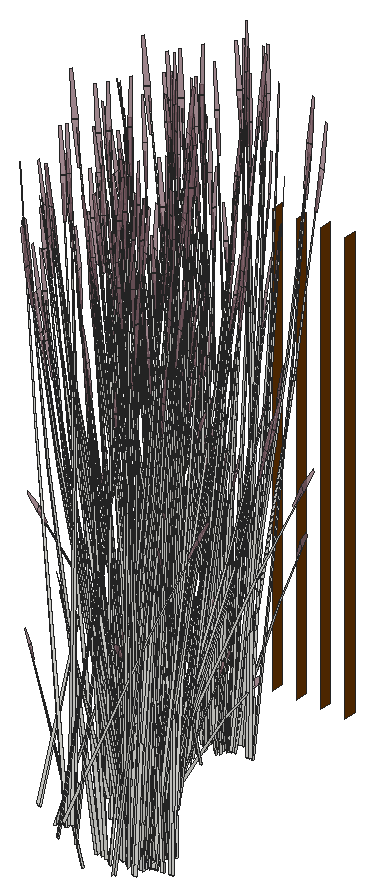
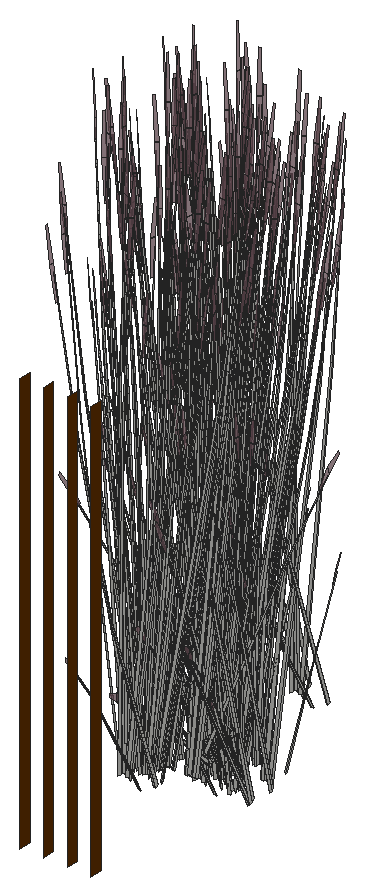
# SketchUp Ruby script. Lengths in inches.
U = 1.inch
M = Sketchup.active_model
def pt(a) = Geom::Point3d.new(a.map { |v| v * U })
def face(e, loops, mat)
  f = e.add_face(loops[0].map { |a| pt(a) })
  loops[1..].each { |l| e.add_face(l.map { |a| pt(a) }).erase! }
  f.material = f.back_material = mat if mat
  f
end
# faces: each face lists its corners as indices into pts; further lists are holes
def faces(e, pts, list, mat = nil) = list.each { |f| face(e, (f[0].is_a?(Array) ? f : [f]).map { |l| l.map { |i| pts[i] } }, mat) }
# xy, xz, yz: faces in a plane at the given z, y or x. An outline is a flat list of corners, or four numbers for a rectangle; further outlines are holes
def ring(l) = l.size == 4 ? [[l[0], l[1]], [l[2], l[1]], [l[2], l[3]], [l[0], l[3]]] : l.each_slice(2).to_a
def flat(e, list, mat, &to3) = list.each { |f| face(e, (f[0].is_a?(Array) ? f : [f]).map { |l| ring(l).map { |u, v| to3.(u, v) } }, mat) }
def xy(e, z, list, mat = nil) = flat(e, list, mat) { |x, y| [x, y, z] }
def xz(e, y, list, mat = nil) = flat(e, list, mat) { |x, z| [x, y, z] }
def yz(e, x, list, mat = nil) = flat(e, list, mat) { |y, z| [x, y, z] }
def lines(e, pts, list) = list.each { |a, b| e.add_line(pt(pts[a]), pt(pts[b])) }
# prism: a flat outline (further loops are holes) pulled along v
def prism(e, loops, v, mat = nil)
  f = face(e, loops, mat); d = Geom::Vector3d.new(v.map { |x| x * U })
  f.pushpull(f.normal.samedirection?(d) ? d.length : -d.length)
end
def box(e, o, s, mat = nil) = prism(e, [[o, [o[0] + s[0], o[1], o[2]], [o[0] + s[0], o[1] + s[1], o[2]], [o[0], o[1] + s[1], o[2]]]], [0, 0, s[2]], mat)
def at(x, y, z, deg = 0) = Geom::Transformation.translation(pt([x, y, z])) * Geom::Transformation.rotation(ORIGIN, Z_AXIS, deg.degrees)
def axes(o, x, y, z) = Geom::Transformation.new([*x, 0, *y, 0, *z, 0, *pt(o).to_a, 1])
def part(name) = M.definitions.add(name)
# library, detail: a bought-in or finely detailed component or shape, given as its bounding box
def library(name, o, s) = part(name).tap { |d| box(d.entities, o, s) }
def detail(e, o, s) = box(e.add_group.entities, o, s)
def put(e, d, t, mat = nil) = e.add_instance(d, t).tap { |i| i.material = mat if mat }
def group(e, t, mat = nil) = e.add_group.tap { |g| g.transformation = t; g.material = mat if mat }.entities
root = M.entities
M.materials.add("C08_Toffee_Ember").color = [102, 51, 0]
M.materials.add("LightPink_Translucent").color = [144, 107, 117]
M.materials["LightPink_Translucent"].alpha = 0.75
c1 = part("blade")
p = [[2.15,0.21,22],[0,0.17,0],[0.09,0.45,0],[2.18,0.31,22],[2.29,0.31,22],[0.38,0.45,0],
  [2.48,0.24,33],[2.49,0.24,33],[2.48,0.22,33]]
faces(c1.entities,p,[[0,1,2,3],[4,5,2,3],[6,3,4,7],[8,0,3,6]])
c2 = part("seeds")
p = [[0.3,-0.1,1.38],[-0.01,-0.03,1.59],[-0.01,-0.03,0.03],[0.14,-0.07,-0.07],[0.29,-0.03,3],[0.15,0.01,3.11]]
faces(c2.entities,p,[[0,1,2,3],[1,0,4,5]],"LightPink_Translucent")
c3 = part("blade with seeds")
put(c3.entities,c1,at(0,0,0))
put(c3.entities,c2,axes([2.4,0.25,30.99],[1.5799,-0.05474,1.17369],[-0.12525,1.92788,0.29478],[-0.07173,-0.02425,1.56792]))
yz(root,675.26,[[360,510,361,546]],"C08_Toffee_Ember")
yz(root,677.28,[[360,510,361,546]],"C08_Toffee_Ember")
yz(root,679.29,[[360,510,361,546]],"C08_Toffee_Ember")
yz(root,681.31,[[360,510,361,546]],"C08_Toffee_Ember")
put(root,c3,axes([678.14,335.36,511.67],[-0.60889,0.28548,-0.4121],[-0.36394,-0.51192,0],[-0.13868,0.06502,1.30728]))
put(root,c3,axes([677.99,341.82,507.1],[-0.60889,-0.28548,-0.4121],[0.36394,-0.51192,0],[-0.13868,-0.06502,1.30728]))
put(root,c3,axes([677,340.73,509.6],[0.60181,0.31483,-0.10093],[-0.34671,0.45593,-0.56021],[-0.17003,0.15849,0.85122]))
put(root,c3,axes([678.71,343.63,512.05],[-0.63528,-0.45956,-0.20909],[0.53456,-0.51604,0.45758],[-0.17107,0.05376,1.39619]))
put(root,c3,axes([677.55,343.19,511.83],[-0.39083,-0.47924,-0.37133],[0.59199,-0.33747,0.17871],[-0.12647,-0.0593,1.19224]))
put(root,c3,axes([678.36,342.17,507.39],[-0.40676,0.57214,0],[-0.68052,-0.31907,-0.42834],[-0.15499,-0.07267,1.3588]))
put(root,c3,axes([677.46,346.24,512.15],[-0.0394,0.18678,1.18691],[-0.57594,0.15636,-0.25526],[-0.13463,-0.24142,0.50747]))
put(root,c3,axes([678.92,349.79,512.21],[-0.65687,0.37907,-0.24149],[-0.43681,-0.53562,-0.41502],[-0.16207,-0.0544,1.32557]))
put(root,c3,axes([678.38,343.53,511.83],[-0.70648,0.03525,-0.37133],[-0.06389,-0.58508,0.17871],[-0.12647,0.0593,1.19224]))
put(root,c3,axes([676.01,342.1,510.11],[0.5741,0.15241,-0.05385],[-0.1766,0.46909,-0.24415],[-0.0939,0.07122,0.8053]))
put(root,c3,axes([676.29,348.96,511.97],[-0.81352,0,0],[0,-0.63814,-0.42834],[0,-0.14534,1.3588]))
put(root,c3,axes([677.43,350.58,511.68],[-0.15283,-0.49751,-0.25712],[0.60696,-0.14127,0.25712],[-0.12236,-0.05737,1.15348]))
put(root,c3,axes([677.29,340.77,509.62],[0.56631,-0.0816,0.29394],[0.14954,0.46647,-0.37948],[-0.16229,0.12529,0.72609]))
put(root,c3,axes([677.62,342.99,507.57],[0.2053,-0.09007,1.18691],[0.50689,0.27159,-0.25526],[-0.15087,0.235,0.50747]))
put(root,c3,axes([675.1,335.53,512.34],[0.59102,-0.10111,0.05401],[0.13587,0.40735,-0.71633],[-0.03747,0.2062,0.64209]))
put(root,c3,axes([677.33,337.86,507.19],[-0.18768,0.46622,-0.03231],[-0.57763,-0.14342,-0.14649],[-0.0877,-0.07626,0.48318]))
put(root,c3,axes([679.35,350.2,511.71],[-0.43821,0.42916,-0.51753],[-0.54436,-0.38915,-0.13583],[-0.1756,0.10706,1.14236]))
put(root,c3,axes([677.61,343.46,512.02],[0.17244,-0.67657,-0.19446],[0.81759,0.11793,0.42555],[-0.14286,-0.09343,1.29846]))
put(root,c3,axes([676.92,348.79,511.93],[-0.60515,0.48003,0.25528],[-0.60552,-0.47498,-0.30288],[-0.02113,-0.13632,1.36855]))
put(root,c3,axes([677.91,343.62,512.17],[-0.12551,0.50956,0.12018],[-0.6132,-0.08845,-0.34318],[-0.1116,-0.05232,1.05198]))
put(root,c3,axes([670.8,347.62,512.15],[-0.23242,-0.01691,1.18691],[-0.23811,-0.45367,-0.25526],[0.28553,-0.12834,0.50747]))
put(root,c3,axes([679.125,345.04,511.67],[-0.60889,0.28548,-0.4121],[-0.36394,-0.51192,0],[-0.13868,0.06502,1.30728]))
put(root,c3,axes([675.52,342.19,511.67],[0,-0.57097,-0.4121],[0.72788,0,0],[0,-0.13004,1.30728]))
put(root,c3,axes([679.64,340.8125,507.64],[-0.65687,0.37907,-0.24149],[-0.43681,-0.53562,-0.41502],[-0.16207,-0.0544,1.32557]))
put(root,c3,axes([679.17,344.89,511.82],[-0.40169,-0.57414,-0.04268],[0.68052,-0.31907,0.42834],[-0.16769,0.05466,1.35813]))
put(root,c3,axes([677.83,342.01,509.35],[-0.46327,-0.38957,0.39842],[0.49199,-0.33598,0.32852],[-0.08546,0.18277,0.82444]))
put(root,c3,axes([679.66,349.96,512.05],[-0.63528,-0.45956,-0.20909],[0.53456,-0.51604,0.45758],[-0.17107,0.05376,1.39619]))
put(root,c3,axes([678.5,349.52,511.83],[-0.39083,-0.47924,-0.37133],[0.59199,-0.33747,0.17871],[-0.12647,-0.0593,1.19224]))
put(root,c3,axes([677.02,339.99,507.39],[-0.81352,0,0],[0,-0.63814,-0.42834],[0,-0.14534,1.3588]))
put(root,c3,axes([678.16,341.61,507.11],[-0.15283,-0.49751,-0.25712],[0.60696,-0.14127,0.25712],[-0.12236,-0.05737,1.15348]))
put(root,c3,axes([677.66,341.97,509.35],[-0.53464,-0.0266,0.05337],[0.01466,-0.40172,0.42015],[-0.05594,0.15388,0.64067]))
put(root,c3,axes([678.98,344.8125,511.68],[-0.60696,-0.14127,-0.25712],[0.15283,-0.49751,0.25712],[-0.12236,0.05737,1.15348]))
put(root,c3,axes([671.23,349.125,511.65],[-0.41902,0.06852,1.17514],[-0.0667,-0.54541,0.06726],[0.29348,-0.08255,0.6687]))
put(root,c3,axes([677.83,342.13,509.18],[-0.4402,0.30062,-0.29394],[-0.41671,-0.34326,0.37948],[-0.0634,0.1744,0.72609]))
put(root,c3,axes([671.6875,348.77,511.24],[-0.034,-0.08668,1.46364],[0.23582,-0.50706,-0.2236],[0.23788,-0.00729,0.24931]))
put(root,c3,axes([679.33,349.86,511.83],[-0.70648,0.03525,-0.37133],[-0.06389,-0.58508,0.17871],[-0.12647,0.0593,1.19224]))
put(root,c3,axes([677.42,342.86,512.21],[-0.73268,-0.27244,-0.24149],[0.35279,-0.57501,-0.41502],[-0.02303,-0.14118,1.32557]))
put(root,c3,axes([680.08,341.23,507.13],[-0.43821,0.42916,-0.51753],[-0.54436,-0.38915,-0.13583],[-0.1756,0.10706,1.14236]))
put(root,c3,axes([676.26,343.2,509.33],[0.07381,-0.03447,1.47228],[0.61004,0.22929,-0.13912],[-0.01434,0.19091,0.26054]))
put(root,c3,axes([677.65,339.82,507.36],[-0.60515,0.48003,0.25528],[-0.60552,-0.47498,-0.30288],[-0.02113,-0.13632,1.36855]))
put(root,c3,axes([676.08,345.2,512.34],[0.59102,-0.10111,0.05401],[0.13587,0.40735,-0.71633],[-0.03747,0.2062,0.64209]))
put(root,c3,axes([678.88,343.37,512.21],[0.07581,0.65151,-0.24149],[-0.7896,0.03939,-0.41502],[-0.13904,0.08678,1.32557]))
put(root,c3,axes([678.69,335.27,511.97],[0.40676,0.57214,0],[-0.68052,0.31907,-0.42834],[-0.15499,0.07267,1.3588]))
put(root,c3,axes([677.1,342.28,511.74],[-0.26718,-0.5855,-0.57963],[0.76964,-0.21087,-0.15213],[-0.02953,-0.19827,1.27944]))
put(root,c3,axes([678.56,349.79,512.02],[0.17244,-0.67657,-0.19446],[0.81759,0.11793,0.42555],[-0.14286,-0.09343,1.29846]))
put(root,c3,axes([680.38,340.99,507.47],[-0.63528,-0.45956,-0.20909],[0.53456,-0.51604,0.45758],[-0.17107,0.05376,1.39619]))
put(root,c3,axes([679.23,340.54,507.26],[-0.39083,-0.47924,-0.37133],[0.59199,-0.33747,0.17871],[-0.12647,-0.0593,1.19224]))
put(root,c3,axes([678.86,349.95,512.17],[-0.12551,0.50956,0.12018],[-0.6132,-0.08845,-0.34318],[-0.1116,-0.05232,1.05198]))
put(root,c3,axes([675.83,342.21,511.68],[0.45414,-0.35624,-0.25712],[0.45414,0.35624,0.25712],[0,-0.11474,1.15348]))
put(root,c3,axes([678.12,341.81,509.85],[-0.01693,0.52814,-0.65454],[-0.71285,-0.03547,0.07899],[-0.07523,0.22375,0.92591]))
put(root,c3,axes([680.08,351.37,511.67],[-0.60889,0.28548,-0.4121],[-0.36394,-0.51192,0],[-0.13868,0.06502,1.30728]))
put(root,c3,axes([676.47,348.53,511.67],[0,-0.57097,-0.4121],[0.72788,0,0],[0,-0.13004,1.30728]))
put(root,c3,axes([677.88,339.9,511.77],[-0.44958,0.32756,-0.03231],[-0.41194,-0.35875,-0.14649],[-0.029,-0.10165,0.48318]))
put(root,c3,axes([680.12,351.22,511.82],[-0.40169,-0.57414,-0.04268],[0.68052,-0.31907,0.42834],[-0.16769,0.05466,1.35813]))
put(root,c3,axes([678.11,343.3,507.72],[-0.01684,-0.3395,0.95334],[0.42072,0.24214,0.70045],[-0.08274,0.16182,0.20998]))
put(root,c3,axes([677.7,343.13,511.96],[0.82229,0.1203,0.37976],[-0.16734,0.67942,0.14902],[-0.12017,-0.06561,1.31851]))
put(root,c3,axes([680.06,340.89,507.26],[-0.70648,0.03525,-0.37133],[-0.06389,-0.58508,0.17871],[-0.12647,0.0593,1.19224]))
put(root,c3,axes([679.93,351.15,511.68],[-0.60696,-0.14127,-0.25712],[0.15283,-0.49751,0.25712],[-0.12236,0.05737,1.15348]))
put(root,c3,axes([678.2,334.92,511.93],[0.81449,0.18558,0.25528],[-0.20377,0.66335,-0.30288],[-0.13481,0.08302,1.36855]))
put(root,c3,axes([678.375,349.1875,512.21],[-0.73268,-0.27244,-0.24149],[0.35279,-0.57501,-0.41502],[-0.02303,-0.14118,1.32557]))
put(root,c3,axes([678.71,341.87,507.48],[0.60889,0.28548,0.4121],[-0.36394,0.51192,0],[-0.13868,-0.06502,1.30728]))
put(root,c3,axes([677.88,342.55,508.22],[0.01429,-0.29475,1.28107],[0.64291,0.15569,0.17703],[-0.0557,0.31414,0.60492]))
put(root,c3,axes([679.28,340.82,507.45],[0.17244,-0.67657,-0.19446],[0.81759,0.11793,0.42555],[-0.14286,-0.09343,1.29846]))
put(root,c3,axes([676.55,335.45,511.24],[0.10529,-0.03107,1.46364],[0.63335,0.17101,-0.2236],[0.01852,0.19274,0.24931]))
put(root,c3,axes([677.03,351.53,512.34],[0.59102,-0.10111,0.05401],[0.13587,0.40735,-0.71633],[-0.03747,0.2062,0.64209]))
put(root,c3,axes([679.58,340.98,507.6],[-0.12551,0.50956,0.12018],[-0.6132,-0.08845,-0.34318],[-0.1116,-0.05232,1.05198]))
put(root,c3,axes([679.83,349.7,512.21],[0.07581,0.65151,-0.24149],[-0.7896,0.03939,-0.41502],[-0.13904,0.08678,1.32557]))
put(root,c3,axes([678.16,344.31,511.82],[-0.65588,-0.25634,0],[0.31565,-0.53263,0],[0,0,1.35047]))
put(root,c3,axes([678.05,348.61,511.74],[-0.26718,-0.5855,-0.57963],[0.76964,-0.21087,-0.15213],[-0.02953,-0.19827,1.27944]))
put(root,c3,axes([679.68,344.95,511.97],[0.40676,0.57214,0],[-0.68052,0.31907,-0.42834],[-0.15499,0.07267,1.3588]))
put(root,c3,axes([680.8,342.4,507.1],[-0.60889,0.28548,-0.4121],[-0.36394,-0.51192,0],[-0.13868,0.06502,1.30728]))
put(root,c3,axes([677.51,340.08,507.48],[0,0.57097,0.4121],[-0.72788,0,0],[0,-0.13004,1.30728]))
put(root,c3,axes([680.84,342.25,507.24],[-0.40169,-0.57414,-0.04268],[0.68052,-0.31907,0.42834],[-0.16769,0.05466,1.35813]))
put(root,c3,axes([676.78,348.54,511.68],[0.45414,-0.35624,-0.25712],[0.45414,0.35624,0.25712],[0,-0.11474,1.15348]))
put(root,c3,axes([678.27,341.99,509.58],[0.46573,0.38364,-0.47077],[-0.49199,0.33598,-0.36465],[-0.07086,0.19492,0.90078]))
put(root,c3,axes([678.83,346.24,511.77],[-0.44958,0.32756,-0.03231],[-0.41194,-0.35875,-0.14649],[-0.029,-0.10165,0.48318]))
put(root,c3,axes([680.66,342.17,507.11],[-0.60696,-0.14127,-0.25712],[0.15283,-0.49751,0.25712],[-0.12236,0.05737,1.15348]))
put(root,c3,axes([679.02,343.5,512.17],[0.48065,0.34305,0.12018],[-0.40092,0.38703,-0.34318],[-0.1116,0.05232,1.05198]))
put(root,c3,axes([678.65,349.47,511.96],[0.82229,0.1203,0.37976],[-0.16734,0.67942,0.14902],[-0.12017,-0.06561,1.31851]))
put(root,c3,axes([678.06,341.7,509.62],[0.4402,-0.30062,0.29394],[0.41671,0.34326,-0.37948],[-0.0634,0.1744,0.72609]))
put(root,c3,axes([679.1,340.21,507.64],[-0.73268,-0.27244,-0.24149],[0.35279,-0.57501,-0.41502],[-0.02303,-0.14118,1.32557]))
put(root,c3,axes([681.01,340.04,507.78],[-0.01777,-0.53759,1.17256],[0.80434,0.13935,0.49647],[-0.19024,0.29416,1.1068]))
put(root,c3,axes([678.85,343.07,511.91],[-0.60515,-0.49144,-0.05089],[0.60552,-0.49174,0],[-0.02113,-0.01716,1.45724]))
put(root,c3,axes([679.18,344.59,511.93],[0.81449,0.18558,0.25528],[-0.20377,0.66335,-0.30288],[-0.13481,0.08302,1.36855]))
put(root,c3,axes([677.78,341.78,509.9],[0.71502,0.02829,-0.11203],[-0.01954,0.53563,-0.62183],[-0.04967,0.20629,0.94486]))
put(root,c3,axes([677.76,342.5625,507.77],[0.59102,-0.10111,0.05401],[0.13587,0.40735,-0.71633],[-0.03747,0.2062,0.64209]))
put(root,c3,axes([680.56,340.73,507.64],[0.07581,0.65151,-0.24149],[-0.7896,0.03939,-0.41502],[-0.13904,0.08678,1.32557]))
put(root,c3,axes([677.63,342.51,511.96],[0.28286,0.63846,0.37976],[-0.80821,0.22202,0.14902],[0.00988,-0.11732,1.31851]))
put(root,c3,axes([677.5,342.43,511.83],[0.31565,-0.51449,-0.37133],[0.65588,0.24761,0.17871],[0,-0.1186,1.19224]))
put(root,c3,axes([678.31,344.09,511.83],[-0.21227,-0.49226,0],[0.60616,-0.17239,0],[0,0,1.28128]))
put(root,c3,axes([678.8,341.44,508.64],[-0.01592,-0.21915,1.42242],[0.69015,0.14538,0.11501],[-0.04269,0.3123,0.60807]))
put(root,c3,axes([677.54,345.125,511.24],[0.10529,-0.03107,1.46364],[0.63335,0.17101,-0.2236],[0.01852,0.19274,0.24931]))
put(root,c3,axes([679.11,350.64,511.82],[-0.65588,-0.25634,0],[0.31565,-0.53263,0],[0,0,1.35047]))
put(root,c3,axes([677.51,339.57,507.11],[0.45414,-0.35624,-0.25712],[0.45414,0.35624,0.25712],[0,-0.11474,1.15348]))
put(root,c3,axes([680.63,351.28,511.97],[0.40676,0.57214,0],[-0.68052,0.31907,-0.42834],[-0.15499,0.07267,1.3588]))
put(root,c3,axes([679.38,340.49,507.38],[0.82229,0.1203,0.37976],[-0.16734,0.67942,0.14902],[-0.12017,-0.06561,1.31851]))
put(root,c3,axes([679.97,349.83,512.17],[0.48065,0.34305,0.12018],[-0.40092,0.38703,-0.34318],[-0.1116,0.05232,1.05198]))
put(root,c3,axes([679.17,340.37,507.68],[-0.31565,0.51449,0.37133],[-0.65588,-0.24761,-0.17871],[0,-0.1186,1.19224]))
put(root,c3,axes([679.17,343.12,511.83],[-0.31565,0.51449,-0.37133],[-0.65588,-0.24761,0.17871],[0,0.1186,1.19224]))
put(root,c3,axes([679.8,349.41,511.91],[-0.60515,-0.49144,-0.05089],[0.60552,-0.49174,0],[-0.02113,-0.01716,1.45724]))
put(root,c3,axes([678.65,342.5625,511.83],[0,-0.66065,0],[0.81352,0,0],[0,0,1.48949]))
put(root,c3,axes([680.13,350.92,511.93],[0.81449,0.18558,0.25528],[-0.20377,0.66335,-0.30288],[-0.13481,0.08302,1.36855]))
put(root,c3,axes([678.95,345.83,511.24],[-0.10912,0.02057,1.46364],[-0.60346,-0.23156,-0.2236],[0.01013,-0.19315,0.24931]))
put(root,c3,axes([678.9375,341.58,507.48],[0.6991,-0.15154,0.14643],[0.17263,0.56398,0.29122],[-0.06235,-0.08217,1.33138]))
put(root,c3,axes([677.89,342.68,512.02],[0.73304,0.27674,0.19974],[-0.35279,0.57501,0.41502],[0,-0.13255,1.3325]))
put(root,c3,axes([679.06,342.83,511.9],[0,0.66033,-0.04679],[-0.81352,0,0],[0,0.02075,1.48875]))
put(root,c3,axes([679.84,341.67,507.25],[-0.65588,-0.25634,0],[0.31565,-0.53263,0],[0,0,1.35047]))
put(root,c3,axes([681.35,342.31,507.39],[0.40676,0.57214,0],[-0.68052,0.31907,-0.42834],[-0.15499,0.07267,1.3588]))
put(root,c3,axes([678.58,348.84,511.96],[0.28286,0.63846,0.37976],[-0.80821,0.22202,0.14902],[0.00988,-0.11732,1.31851]))
put(root,c3,axes([678.45,348.76,511.83],[0.31565,-0.51449,-0.37133],[0.65588,0.24761,0.17871],[0,-0.1186,1.19224]))
put(root,c3,axes([679.26,350.42,511.83],[-0.21227,-0.49226,0],[0.60616,-0.17239,0],[0,0,1.28128]))
put(root,c3,axes([678.67,344.1,511.9],[0.28286,0.65594,-0.0499],[-0.80821,0.22985,0],[0.00988,0.02291,1.42904]))
put(root,c3,axes([679.28,342.56,509.625],[-0.64106,-0.14927,0.44225],[0.21921,-0.49074,0.36465],[0.03852,0.19299,0.91512]))
put(root,c3,axes([678.49,351.46,511.24],[0.10529,-0.03107,1.46364],[0.63335,0.17101,-0.2236],[0.01852,0.19274,0.24931]))
put(root,c3,axes([679.11,342.59,509.35],[-0.47939,0.19405,0.05337],[-0.23464,-0.35385,0.42015],[0.0463,0.15598,0.64067]))
put(root,c3,axes([678.55,333.59,511.74],[0.23855,0.52277,-0.57446],[-0.68718,0.18827,-0.15077],[0.02637,0.17702,1.26801]))
put(root,c3,axes([681.02,341.61,507.48],[0.18794,-0.56744,0.14643],[0.68774,0.16058,0.29122],[-0.1188,0.00276,1.33138]))
put(root,c3,axes([680.7,340.86,507.6],[0.48065,0.34305,0.12018],[-0.40092,0.38703,-0.34318],[-0.1116,0.05232,1.05198]))
put(root,c3,axes([676.99,340.59,511.97],[-0.40676,-0.57214,0],[0.68052,-0.31907,-0.42834],[0.15499,-0.07267,1.3588]))
put(root,c3,axes([681.01,343.24,511.83],[-0.81312,-0.00457,-0.0413],[0,-0.63814,0.41452],[-0.02555,0.14527,1.31432]))
put(root,c3,axes([680.53,340.43,507.33],[-0.60515,-0.49144,-0.05089],[0.60552,-0.49174,0],[-0.02113,-0.01716,1.45724]))
put(root,c3,axes([680.6875,340.6,507.68],[0.70648,-0.03525,0.37133],[0.06389,0.58508,-0.17871],[-0.12647,0.0593,1.19224]))
put(root,c3,axes([680.12,349.45,511.83],[-0.31565,0.51449,-0.37133],[-0.65588,-0.24761,0.17871],[0,0.1186,1.19224]))
put(root,c3,axes([680.86,341.95,507.36],[0.81449,0.18558,0.25528],[-0.20377,0.66335,-0.30288],[-0.13481,0.08302,1.36855]))
put(root,c3,axes([681.21,341.91,507.48],[0.60889,-0.28548,0.4121],[0.36394,0.51192,0],[-0.13868,0.06502,1.30728]))
put(root,c3,axes([678.26,342.15,511.96],[-0.53943,0.51816,0.37976],[-0.64086,-0.4574,0.14902],[0.13005,-0.05171,1.31851]))
put(root,c3,axes([679.31,339.87,507.38],[0.28286,0.63846,0.37976],[-0.80821,0.22202,0.14902],[0.00988,-0.11732,1.31851]))
put(root,c3,axes([679.19,342.96,511.84],[0.45414,0.3688,0],[-0.45414,0.3688,0],[0,0,1.40491]))
put(root,c3,axes([679.6,348.89,511.83],[0,-0.66065,0],[0.81352,0,0],[0,0,1.48949]))
put(root,c3,axes([679.18,339.79,507.26],[0.31565,-0.51449,-0.37133],[0.65588,0.24761,0.17871],[0,-0.1186,1.19224]))
put(root,c3,axes([678.91,344.32,511.83],[0.65588,0.25634,0],[-0.31565,0.53263,0],[0,0,1.45212]))
put(root,c3,axes([679.99,341.45,507.25],[-0.21227,-0.49226,0],[0.60616,-0.17239,0],[0,0,1.28128]))
put(root,c3,axes([678.84,349.01,512.02],[0.73304,0.27674,0.19974],[-0.35279,0.57501,0.41502],[0,-0.13255,1.3325]))
put(root,c3,axes([679.22,342.48,506.66],[0.10529,-0.03107,1.46364],[0.63335,0.17101,-0.2236],[0.01852,0.19274,0.24931]))
put(root,c3,axes([680.01,349.16,511.9],[0,0.66033,-0.04679],[-0.81352,0,0],[0,0.02075,1.48875]))
put(root,c3,axes([679.36,342.66,509.18],[-0.19614,0.43908,-0.29394],[-0.57222,-0.12807,0.37948],[0.05247,0.17678,0.72609]))
put(root,c3,axes([678.97,342.41,511.98],[-0.82229,-0.1203,0.40835],[0.16734,-0.67942,0.16024],[0.12017,0.06561,1.41775]))
put(root,c3,axes([680.16,333.67,511.67],[0,0.57097,-0.4121],[-0.72788,0,0],[0,0.13004,1.30728]))
put(root,c3,axes([679.62,350.4375,511.9],[0.28286,0.65594,-0.0499],[-0.80821,0.22985,0],[0.00988,0.02291,1.42904]))
put(root,c3,axes([680.84,343.34,511.68],[-0.45414,0.35624,-0.25712],[-0.45414,-0.35624,0.25712],[0,0.11474,1.15348]))
put(root,c3,axes([679.54,343.27,511.74],[0.23855,0.52277,-0.57446],[-0.68718,0.18827,-0.15077],[0.02637,0.17702,1.26801]))
put(root,c3,axes([679.2,342.71,511.83],[0.72788,0,0],[0,0.59111,0],[0,0,1.48078]))
put(root,c3,axes([680.84,340.48,507.26],[-0.31565,0.51449,-0.37133],[-0.65588,-0.24761,0.17871],[0,0.1186,1.19224]))
put(root,c3,axes([677.94,346.92,511.97],[-0.40676,-0.57214,0],[0.68052,-0.31907,-0.42834],[0.15499,-0.07267,1.3588]))
put(root,c3,axes([681.96,349.58,511.83],[-0.81312,-0.00457,-0.0413],[0,-0.63814,0.41452],[-0.02555,0.14527,1.31432]))
put(root,c3,axes([677.79,342.17,512.21],[-0.07581,-0.65151,-0.24149],[0.7896,-0.03939,-0.41502],[0.13904,-0.08678,1.32557]))
put(root,c3,axes([679.45,342.65,512.17],[0.60616,-0.16651,0.12018],[0.21227,0.47548,-0.34318],[0,0.10465,1.05198]))
put(root,c3,axes([678.95,343.4375,509.34],[0.08247,0.09194,1.45204],[0.66552,0.03612,-0.22964],[0.06692,0.20277,0.11645]))
put(root,c3,axes([682.09,340.16,507.48],[-0.51116,-0.4159,0.14643],[0.51512,-0.4034,0.29122],[-0.05645,0.08494,1.33138]))
put(root,c3,axes([680.33,339.92,507.25],[0,-0.66065,0],[0.81352,0,0],[0,0,1.48949]))
put(root,c3,axes([679.57,340.04,507.44],[0.73304,0.27674,0.19974],[-0.35279,0.57501,0.41502],[0,-0.13255,1.3325]))
put(root,c3,axes([680.73,340.19,507.33],[0,0.66033,-0.04679],[-0.81352,0,0],[0,0.02075,1.48875]))
put(root,c3,axes([679.33,339.66,507.68],[-0.70648,0.03525,0.37133],[-0.06389,-0.58508,-0.17871],[0.12647,-0.0593,1.19224]))
put(root,c3,axes([679.29,342.2,509.62],[0.19614,-0.43908,0.29394],[0.57222,0.12807,-0.37948],[0.05247,0.17678,0.72609]))
put(root,c3,axes([679.25,342.6875,512.21],[0.73268,0.27244,-0.24149],[-0.35279,0.57501,-0.41502],[0.02303,0.14118,1.32557]))
put(root,c3,axes([679.21,348.48,511.96],[-0.53943,0.51816,0.37976],[-0.64086,-0.4574,0.14902],[0.13005,-0.05171,1.31851]))
put(root,c3,axes([680.14,349.3,511.84],[0.45414,0.3688,0],[-0.45414,0.3688,0],[0,0,1.40491]))
put(root,c3,axes([679.86,350.65,511.83],[0.65588,0.25634,0],[-0.31565,0.53263,0],[0,0,1.45212]))
put(root,c3,axes([679,338.65,507.48],[-0.18794,0.56744,0.14643],[-0.68774,-0.16058,0.29122],[0.1188,-0.00276,1.33138]))
put(root,c3,axes([677.6875,340.73,511.68],[0.60696,0.14127,-0.25712],[-0.15283,0.49751,0.25712],[0.12236,-0.05737,1.15348]))
put(root,c3,axes([680.35,341.46,507.33],[0.28286,0.65594,-0.0499],[-0.80821,0.22985,0],[0.00988,0.02291,1.42904]))
put(root,c3,axes([679.92,348.74,511.98],[-0.82229,-0.1203,0.40835],[0.16734,-0.67942,0.16024],[0.12017,0.06561,1.41775]))
put(root,c3,axes([681.15,343.35,511.67],[0,0.57097,-0.4121],[-0.72788,0,0],[0,0.13004,1.30728]))
put(root,c3,axes([677.54,340.5,511.67],[0.60889,-0.28548,-0.4121],[0.36394,0.51192,0],[0.13868,-0.06502,1.30728]))
put(root,c3,axes([681.79,349.67,511.68],[-0.45414,0.35624,-0.25712],[-0.45414,-0.35624,0.25712],[0,0.11474,1.15348]))
put(root,c3,axes([679.41,342.26,509.56],[0.31051,0.46426,-0.58968],[-0.63919,0.25873,0.07116],[0.07261,0.22432,0.83415]))
put(root,c3,axes([682.68,340.6,507.25],[-0.81312,-0.00457,-0.0413],[0,-0.63814,0.41452],[-0.02555,0.14527,1.31432]))
put(root,c3,axes([678.76,341.92,512.17],[0.12551,-0.50956,0.12018],[0.6132,0.08845,-0.34318],[0.1116,0.05232,1.05198]))
put(root,c3,axes([677.93,334.68,512.15],[0.01148,-0.18927,1.18691],[0.54864,-0.21141,-0.25526],[0.16937,0.22654,0.50747]))
put(root,c3,axes([681.08,338.68,507.48],[-0.6991,0.15154,0.14643],[-0.17263,-0.56398,0.29122],[0.06235,0.08217,1.33138]))
put(root,c3,axes([680.49,349.6,511.74],[0.23855,0.52277,-0.57446],[-0.68718,0.18827,-0.15077],[0.02637,0.17702,1.26801]))
put(root,c3,axes([680.15,349.04,511.83],[0.72788,0,0],[0,0.59111,0],[0,0,1.48078]))
put(root,c3,axes([678.74,348.5,512.21],[-0.07581,-0.65151,-0.24149],[0.7896,-0.03939,-0.41502],[0.13904,-0.08678,1.32557]))
put(root,c3,axes([680.0625,343.76,510.11],[0.44958,-0.32756,-0.05385],[0.41194,0.35875,-0.24415],[0.029,0.10165,0.8053]))
put(root,c3,axes([680.4,348.98,512.17],[0.60616,-0.16651,0.12018],[0.21227,0.47548,-0.34318],[0,0.10465,1.05198]))
put(root,c3,axes([679.94,339.51,507.38],[-0.53943,0.51816,0.37976],[-0.64086,-0.4574,0.14902],[0.13005,-0.05171,1.31851]))
put(root,c3,axes([680.86,340.32,507.26],[0.45414,0.3688,0],[-0.45414,0.3688,0],[0,0,1.40491]))
put(root,c3,axes([680.86,339.89,507.68],[0.31565,-0.51449,0.37133],[0.65588,0.24761,-0.17871],[0,0.1186,1.19224]))
put(root,c3,axes([680.58,341.68,507.25],[0.65588,0.25634,0],[-0.31565,0.53263,0],[0,0,1.45212]))
put(root,c3,axes([679.1,344.02,511.8125],[0.68303,-0.19373,-0.15934],[0.24001,0.55805,0.00007],[0.07539,-0.02141,1.44335]))
put(root,c3,axes([679.65,342.36,509.31],[0.63954,0.14313,-0.42412],[-0.21921,0.49074,-0.32852],[0.05864,0.19758,0.81151]))
put(root,c3,axes([680.2,349.02,512.21],[0.73268,0.27244,-0.24149],[-0.35279,0.57501,-0.41502],[0.02303,0.14118,1.32557]))
put(root,c3,axes([679.1,342.38,509.6],[0.63664,-0.26583,-0.10093],[0.31286,0.47181,-0.56021],[0.084,0.19882,0.85122]))
put(root,c3,axes([680.64,339.77,507.4],[-0.82229,-0.1203,0.40835],[0.16734,-0.67942,0.16024],[0.12017,0.06561,1.41775]))
put(root,c3,axes([678.64,347.0625,511.68],[0.60696,0.14127,-0.25712],[-0.15283,0.49751,0.25712],[0.12236,-0.05737,1.15348]))
put(root,c3,axes([682.51,340.7,507.11],[-0.45414,0.35624,-0.25712],[-0.45414,-0.35624,0.25712],[0,0.11474,1.15348]))
put(root,c3,axes([680.33,346.46,512.15],[-0.18493,0.11557,1.18691],[-0.55384,-0.20228,-0.25526],[0.10266,-0.25157,0.50747]))
put(root,c3,axes([679.12,342.36,511.83],[0.39083,0.47924,-0.37133],[-0.59199,0.33747,0.17871],[0.12647,0.0593,1.19224]))
put(root,c3,axes([681.21,340.63,507.16],[0.23855,0.52277,-0.57446],[-0.68718,0.18827,-0.15077],[0.02637,0.17702,1.26801]))
put(root,c3,axes([680.88,340.07,507.25],[0.72788,0,0],[0,0.59111,0],[0,0,1.48078]))
put(root,c3,axes([682.1,349.68,511.67],[0,0.57097,-0.4121],[-0.72788,0,0],[0,0.13004,1.30728]))
put(root,c3,axes([678.49,346.84,511.67],[0.60889,-0.28548,-0.4121],[0.36394,0.51192,0],[0.13868,-0.06502,1.30728]))
put(root,c3,axes([680.18,339.42,507.68],[-0.39083,-0.47924,0.37133],[0.59199,-0.33747,-0.17871],[0.12647,0.0593,1.19224]))
put(root,c3,axes([679.47,339.53,507.64],[-0.07581,-0.65151,-0.24149],[0.7896,-0.03939,-0.41502],[0.13904,-0.08678,1.32557]))
put(root,c3,axes([679.71,348.26,512.17],[0.12551,-0.50956,0.12018],[0.6132,0.08845,-0.34318],[0.1116,0.05232,1.05198]))
put(root,c3,axes([681.13,340.01,507.6],[0.60616,-0.16651,0.12018],[0.21227,0.47548,-0.34318],[0,0.10465,1.05198]))
put(root,c3,axes([678.92,344.36,512.15],[0.01148,-0.18927,1.18691],[0.54864,-0.21141,-0.25526],[0.16937,0.22654,0.50747]))
put(root,c3,axes([678.26,341.68,511.71],[0.43821,-0.42916,-0.51753],[0.54436,0.38915,-0.13583],[0.1756,-0.10706,1.14236]))
put(root,c3,axes([680.92,340.05,507.64],[0.73268,0.27244,-0.24149],[-0.35279,0.57501,-0.41502],[0.02303,0.14118,1.32557]))
put(root,c3,axes([679.36,338.09,507.11],[0.60696,0.14127,-0.25712],[-0.15283,0.49751,0.25712],[0.12236,-0.05737,1.15348]))
put(root,c3,axes([680.06,350.35,511.8125],[0.68303,-0.19373,-0.15934],[0.24001,0.55805,0.00007],[0.07539,-0.02141,1.44335]))
put(root,c3,axes([680.1875,341.29,511.68],[0.15283,0.49751,-0.25712],[-0.60696,0.14127,0.25712],[0.12236,0.05737,1.15348]))
